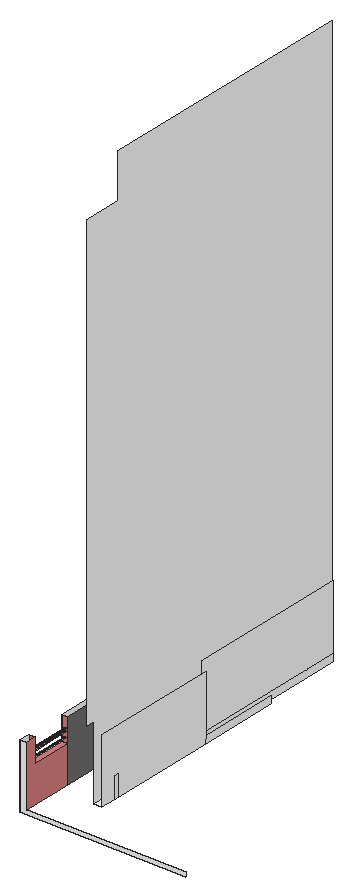
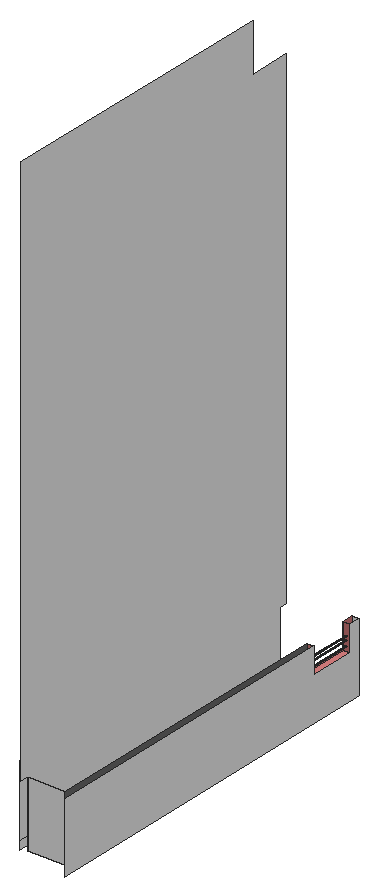
# SketchUp Ruby script. Lengths in inches.
U = 1.inch
M = Sketchup.active_model
def pt(a) = Geom::Point3d.new(a.map { |v| v * U })
def face(e, loops, mat)
  f = e.add_face(loops[0].map { |a| pt(a) })
  loops[1..].each { |l| e.add_face(l.map { |a| pt(a) }).erase! }
  f.material = f.back_material = mat if mat
  f
end
# faces: each face lists its corners as indices into pts; further lists are holes
def faces(e, pts, list, mat = nil) = list.each { |f| face(e, (f[0].is_a?(Array) ? f : [f]).map { |l| l.map { |i| pts[i] } }, mat) }
# xy, xz, yz: faces in a plane at the given z, y or x. An outline is a flat list of corners, or four numbers for a rectangle; further outlines are holes
def ring(l) = l.size == 4 ? [[l[0], l[1]], [l[2], l[1]], [l[2], l[3]], [l[0], l[3]]] : l.each_slice(2).to_a
def flat(e, list, mat, &to3) = list.each { |f| face(e, (f[0].is_a?(Array) ? f : [f]).map { |l| ring(l).map { |u, v| to3.(u, v) } }, mat) }
def xy(e, z, list, mat = nil) = flat(e, list, mat) { |x, y| [x, y, z] }
def xz(e, y, list, mat = nil) = flat(e, list, mat) { |x, z| [x, y, z] }
def yz(e, x, list, mat = nil) = flat(e, list, mat) { |y, z| [x, y, z] }
def lines(e, pts, list) = list.each { |a, b| e.add_line(pt(pts[a]), pt(pts[b])) }
# prism: a flat outline (further loops are holes) pulled along v
def prism(e, loops, v, mat = nil)
  f = face(e, loops, mat); d = Geom::Vector3d.new(v.map { |x| x * U })
  f.pushpull(f.normal.samedirection?(d) ? d.length : -d.length)
end
def box(e, o, s, mat = nil) = prism(e, [[o, [o[0] + s[0], o[1], o[2]], [o[0] + s[0], o[1] + s[1], o[2]], [o[0], o[1] + s[1], o[2]]]], [0, 0, s[2]], mat)
def at(x, y, z, deg = 0) = Geom::Transformation.translation(pt([x, y, z])) * Geom::Transformation.rotation(ORIGIN, Z_AXIS, deg.degrees)
def axes(o, x, y, z) = Geom::Transformation.new([*x, 0, *y, 0, *z, 0, *pt(o).to_a, 1])
def part(name) = M.definitions.add(name)
# library, detail: a bought-in or finely detailed component or shape, given as its bounding box
def library(name, o, s) = part(name).tap { |d| box(d.entities, o, s) }
def detail(e, o, s) = box(e.add_group.entities, o, s)
def put(e, d, t, mat = nil) = e.add_instance(d, t).tap { |i| i.material = mat if mat }
def group(e, t, mat = nil) = e.add_group.tap { |g| g.transformation = t; g.material = mat if mat }.entities
root = M.entities
M.materials.add("[Color M00]").color = [255, 255, 255]
M.materials.add("[Color M05]").color = [114, 114, 114]
M.materials.add("[Tile Various Tan]").color = [221, 130, 130]
xy(root,5.5625,[[61.5,83.25,74.88,129.875]],"[Color M00]")
xy(root,61.5625,[[0,37.7,9.51,100.01]],"[Tile Various Tan]")
xz(root,21.25,[[0,0,251.02,0,251.02,5.5625,9.51,5.5625,9.51,97.5625,0,97.5625]],"[Color M00]")
xz(root,37.7,[[[0,61.5625,9.51,97.5625],[4.83,93.79,5.02,93.8,5.21,93.86,5.375,93.96,5.51,94.11,5.6,94.28,5.64,94.47,5.63,94.67,5.57,94.85,5.47,95.02,5.32,95.15,5.15,95.24,4.96,95.28,4.76,95.27,4.58,95.22,4.41,95.11,4.28,94.97,4.1875,94.79,4.15,94.6,4.15,94.41,4.21,94.22,4.32,94.05,4.46,93.92,4.64,93.83],[4.83,86.79,5.02,86.8,5.21,86.86,5.375,86.96,5.51,87.11,5.6,87.28,5.64,87.47,5.63,87.67,5.57,87.85,5.47,88.02,5.32,88.15,5.15,88.24,4.96,88.28,4.76,88.27,4.58,88.22,4.41,88.11,4.28,87.97,4.1875,87.79,4.15,87.6,4.15,87.41,4.21,87.22,4.32,87.05,4.46,86.92,4.64,86.83],[4.83,80.23,5.02,80.24,5.21,80.29,5.375,80.4,5.51,80.54,5.6,80.72,5.64,80.91,5.63,81.1,5.57,81.29,5.47,81.46,5.32,81.59,5.15,81.68,4.96,81.72,4.76,81.71,4.58,81.65,4.41,81.55,4.28,81.4,4.1875,81.23,4.15,81.04,4.15,80.84,4.21,80.66,4.32,80.49,4.46,80.36,4.64,80.27],[4.83,75.04,5.02,75.05,5.21,75.11,5.375,75.21,5.51,75.36,5.6,75.53,5.64,75.72,5.63,75.92,5.57,76.1,5.47,76.27,5.32,76.4,5.15,76.49,4.96,76.53,4.76,76.52,4.58,76.47,4.41,76.36,4.28,76.22,4.1875,76.04,4.15,75.85,4.15,75.66,4.21,75.47,4.32,75.3,4.46,75.17,4.64,75.08],[4.83,67.29,5.02,67.3,5.21,67.36,5.375,67.46,5.51,67.61,5.6,67.78,5.64,67.97,5.63,68.17,5.57,68.35,5.47,68.52,5.32,68.65,5.15,68.74,4.96,68.78,4.76,68.77,4.58,68.72,4.41,68.61,4.28,68.47,4.1875,68.29,4.15,68.1,4.15,67.91,4.21,67.72,4.32,67.55,4.46,67.42,4.64,67.33]]],"[Tile Various Tan]")
xz(root,100.01,[[[0,61.5625,9.51,97.5625],[4.83,93.79,4.64,93.83,4.46,93.92,4.32,94.05,4.21,94.22,4.15,94.41,4.15,94.6,4.1875,94.79,4.28,94.97,4.41,95.11,4.58,95.22,4.76,95.27,4.96,95.28,5.15,95.24,5.32,95.15,5.47,95.02,5.57,94.85,5.63,94.67,5.64,94.47,5.6,94.28,5.51,94.11,5.375,93.96,5.21,93.86,5.02,93.8],[4.83,86.79,4.64,86.83,4.46,86.92,4.32,87.05,4.21,87.22,4.15,87.41,4.15,87.6,4.1875,87.79,4.28,87.97,4.41,88.11,4.58,88.22,4.76,88.27,4.96,88.28,5.15,88.24,5.32,88.15,5.47,88.02,5.57,87.85,5.63,87.67,5.64,87.47,5.6,87.28,5.51,87.11,5.375,86.96,5.21,86.86,5.02,86.8],[4.83,80.23,4.64,80.27,4.46,80.36,4.32,80.49,4.21,80.66,4.15,80.84,4.15,81.04,4.1875,81.23,4.28,81.4,4.41,81.55,4.58,81.65,4.76,81.71,4.96,81.72,5.15,81.68,5.32,81.59,5.47,81.46,5.57,81.29,5.63,81.1,5.64,80.91,5.6,80.72,5.51,80.54,5.375,80.4,5.21,80.29,5.02,80.24],[4.83,75.04,4.64,75.08,4.46,75.17,4.32,75.3,4.21,75.47,4.15,75.66,4.15,75.85,4.1875,76.04,4.28,76.22,4.41,76.36,4.58,76.47,4.76,76.52,4.96,76.53,5.15,76.49,5.32,76.4,5.47,76.27,5.57,76.1,5.63,75.92,5.64,75.72,5.6,75.53,5.51,75.36,5.375,75.21,5.21,75.11,5.02,75.05],[4.83,67.29,4.64,67.33,4.46,67.42,4.32,67.55,4.21,67.72,4.15,67.91,4.15,68.1,4.1875,68.29,4.28,68.47,4.41,68.61,4.58,68.72,4.76,68.77,4.96,68.78,5.15,68.74,5.32,68.65,5.47,68.52,5.57,68.35,5.63,68.17,5.64,67.97,5.6,67.78,5.51,67.61,5.375,67.46,5.21,67.36,5.02,67.3]]],"[Tile Various Tan]")
xz(root,279.08,[[69.2,5.5625,74.88,16.29]],"[Color M00]")
xz(root,523,[[9.51,5.5625,61.5,97.5625]],"[Color M00]")
yz(root,0,[[21.25,0,21.25,97.5625,37.7,97.5625,37.7,61.5625,100.01,61.5625,100.01,97.5625,535.125,97.5625,535.125,0]],"[Color M00]")
yz(root,4.15,[[37.7,67.91,100.01,68.1],[37.7,75.66,100.01,75.85],[37.7,80.84,100.01,81.04]],"[Color M00]")
yz(root,9.51,[[100.01,5.5625,523,97.5625]],"[Color M05]")
yz(root,9.51,[[21.25,5.5625,100.01,5.5625,100.01,61.5625,37.7,61.5625,37.7,97.5625,21.25,97.5625]],"[Tile Various Tan]")
yz(root,61.5,[[83.25,5.5625,83.25,116.25,71.125,116.25,71.125,805.18,129.875,805.18,129.875,873.0625,535.125,873.0625,535.125,97.5625,523,97.5625,523,5.5625]],"[Color M00]")
yz(root,69.2,[[279.08,5.5625,527.42,16.29],[279.08,16.29,527.42,116.6875]],"[Color M00]")
yz(root,74.88,[[83.25,5.5625,106.0625,5.5625,106.0625,37.95,113.875,37.95,113.875,5.5625,279.08,5.5625,279.08,103.5,83.25,103.5],[106.0625,5.5625,113.875,37.95],[279.08,5.5625,403.25,16.29]],"[Color M00]")
p = [[4.46,100.01,67.42],[4.64,100.01,67.33],[4.64,37.7,67.33],[4.46,37.7,67.42],[4.83,100.01,67.29],[4.83,37.7,67.29],
  [5.02,100.01,67.3],[5.02,37.7,67.3],[5.21,100.01,67.36],[5.21,37.7,67.36],[4.32,100.01,67.55],[4.32,37.7,67.55],
  [5.375,100.01,67.46],[5.375,37.7,67.46],[5.51,100.01,67.61],[5.51,37.7,67.61],[4.21,100.01,67.72],[4.21,37.7,67.72],
  [5.6,100.01,67.78],[5.6,37.7,67.78],[4.15,100.01,67.91],[4.15,37.7,67.91],[5.64,100.01,67.97],[5.64,37.7,67.97],
  [5.63,100.01,68.17],[5.63,37.7,68.17],[4.1875,100.01,68.29],[4.15,100.01,68.1],[4.15,37.7,68.1],[4.1875,37.7,68.29],
  [5.57,100.01,68.35],[5.57,37.7,68.35],[4.28,100.01,68.47],[4.28,37.7,68.47],[5.47,100.01,68.52],[5.47,37.7,68.52],
  [4.41,100.01,68.61],[4.41,37.7,68.61],[5.32,100.01,68.65],[5.32,37.7,68.65],[4.58,100.01,68.72],[4.58,37.7,68.72],
  [4.76,100.01,68.77],[4.76,37.7,68.77],[5.15,100.01,68.74],[4.96,100.01,68.78],[4.96,37.7,68.78],[5.15,37.7,68.74],
  [4.64,100.01,75.08],[4.83,100.01,75.04],[4.83,37.7,75.04],[4.64,37.7,75.08],[5.02,100.01,75.05],[5.02,37.7,75.05],
  [5.21,100.01,75.11],[5.21,37.7,75.11],[4.46,100.01,75.17],[4.46,37.7,75.17],[5.375,100.01,75.21],[5.375,37.7,75.21],
  [4.32,100.01,75.3],[4.32,37.7,75.3],[5.51,100.01,75.36],[5.51,37.7,75.36],[4.21,100.01,75.47],[4.21,37.7,75.47],
  [5.6,100.01,75.53],[5.6,37.7,75.53],[4.15,100.01,75.66],[4.15,37.7,75.66],[5.64,100.01,75.72],[5.64,37.7,75.72],
  [5.63,100.01,75.92],[5.63,37.7,75.92],[4.1875,100.01,76.04],[4.15,100.01,75.85],[4.15,37.7,75.85],[4.1875,37.7,76.04],
  [5.57,100.01,76.1],[5.57,37.7,76.1],[4.28,100.01,76.22],[4.28,37.7,76.22],[5.47,100.01,76.27],[5.47,37.7,76.27],
  [4.41,100.01,76.36],[4.41,37.7,76.36],[5.32,100.01,76.4],[5.32,37.7,76.4],[4.58,100.01,76.47],[4.58,37.7,76.47],
  [5.15,100.01,76.49],[5.15,37.7,76.49],[4.76,100.01,76.52],[4.76,37.7,76.52],[4.96,100.01,76.53],[4.96,37.7,76.53],
  [4.64,100.01,80.27],[4.83,100.01,80.23],[4.83,37.7,80.23],[4.64,37.7,80.27],[5.02,100.01,80.24],[5.02,37.7,80.24],
  [5.21,100.01,80.29],[5.21,37.7,80.29],[4.46,100.01,80.36],[4.46,37.7,80.36],[5.375,100.01,80.4],[5.375,37.7,80.4],
  [4.32,100.01,80.49],[4.32,37.7,80.49],[5.51,100.01,80.54],[5.51,37.7,80.54],[4.21,100.01,80.66],[4.21,37.7,80.66],
  [5.6,100.01,80.72],[5.6,37.7,80.72],[4.15,100.01,80.84],[4.15,37.7,80.84],[5.64,100.01,80.91],[5.64,37.7,80.91],
  [5.63,100.01,81.1],[5.63,37.7,81.1],[4.1875,100.01,81.23],[4.15,100.01,81.04],[4.15,37.7,81.04],[4.1875,37.7,81.23],
  [5.57,100.01,81.29],[5.57,37.7,81.29],[4.28,100.01,81.4],[4.28,37.7,81.4],[5.47,100.01,81.46],[5.47,37.7,81.46],
  [4.41,100.01,81.55],[4.41,37.7,81.55],[4.58,100.01,81.65],[4.58,37.7,81.65],[5.32,100.01,81.59],[5.32,37.7,81.59],
  [5.15,100.01,81.68],[5.15,37.7,81.68],[4.76,100.01,81.71],[4.76,37.7,81.71],[4.96,100.01,81.72],[4.96,37.7,81.72]]
faces(root,p,[[0,1,2,3],[1,4,5,2],[4,6,7,5],[6,8,9,7],[10,0,3,11],[8,12,13,9],[12,14,15,13],[16,10,11,17],
  [14,18,19,15],[20,16,17,21],[18,22,23,19],[22,24,25,23],[26,27,28,29],[24,30,31,25],[32,26,29,33],[30,34,35,31],
  [36,32,33,37],[34,38,39,35],[40,36,37,41],[42,40,41,43],[44,45,46,47],[38,44,47,39],[45,42,43,46],[48,49,50,51],
  [49,52,53,50],[52,54,55,53],[56,48,51,57],[54,58,59,55],[60,56,57,61],[58,62,63,59],[64,60,61,65],[62,66,67,63],
  [68,64,65,69],[66,70,71,67],[70,72,73,71],[74,75,76,77],[72,78,79,73],[80,74,77,81],[78,82,83,79],[84,80,81,85],
  [82,86,87,83],[88,84,85,89],[86,90,91,87],[92,88,89,93],[94,92,93,95],[90,94,95,91],[96,97,98,99],[97,100,101,98],
  [100,102,103,101],[104,96,99,105],[102,106,107,103],[108,104,105,109],[106,110,111,107],[112,108,109,113],[110,114,115,111],[116,112,113,117],
  [114,118,119,115],[118,120,121,119],[122,123,124,125],[120,126,127,121],[128,122,125,129],[126,130,131,127],[132,128,129,133],[134,132,133,135],
  [130,136,137,131],[136,138,139,137],[140,134,135,141],[142,140,141,143],[138,142,143,139]],"[Color M00]")
